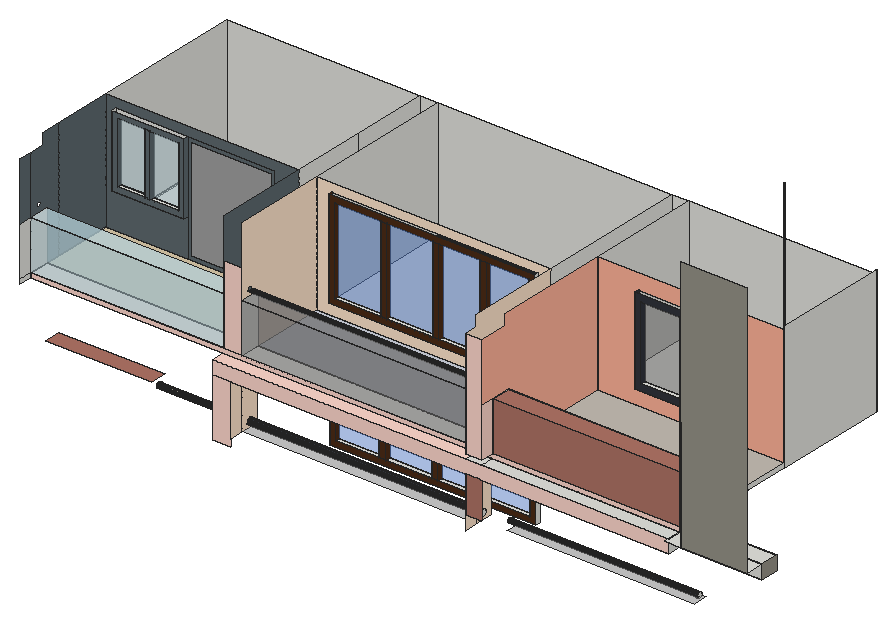
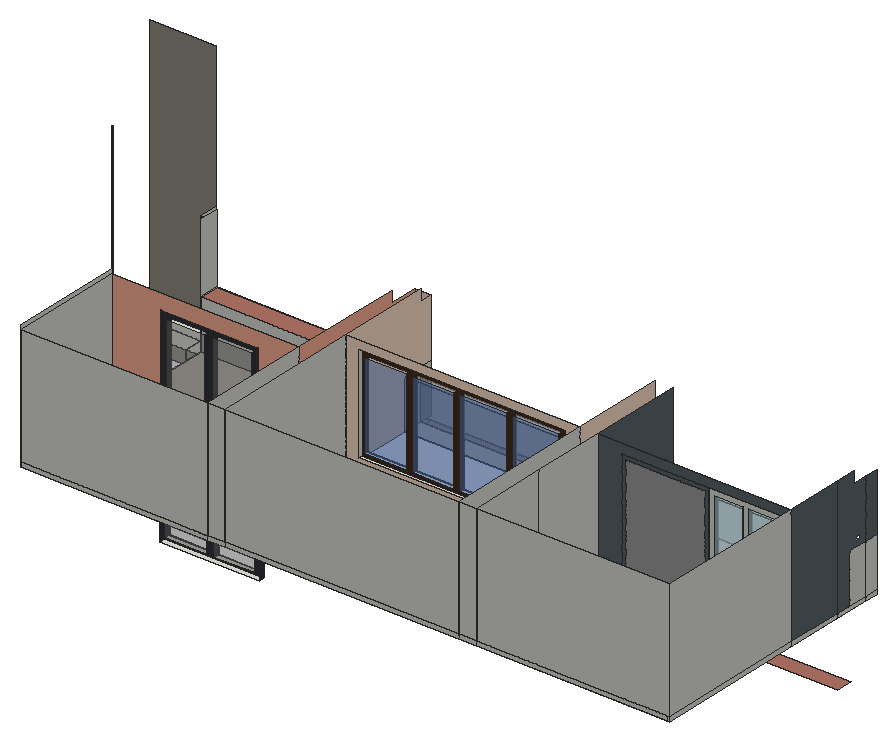
# SketchUp Ruby script. Lengths in inches.
U = 1.inch
M = Sketchup.active_model
def pt(a) = Geom::Point3d.new(a.map { |v| v * U })
def face(e, loops, mat)
  f = e.add_face(loops[0].map { |a| pt(a) })
  loops[1..].each { |l| e.add_face(l.map { |a| pt(a) }).erase! }
  f.material = f.back_material = mat if mat
  f
end
# faces: each face lists its corners as indices into pts; further lists are holes
def faces(e, pts, list, mat = nil) = list.each { |f| face(e, (f[0].is_a?(Array) ? f : [f]).map { |l| l.map { |i| pts[i] } }, mat) }
# xy, xz, yz: faces in a plane at the given z, y or x. An outline is a flat list of corners, or four numbers for a rectangle; further outlines are holes
def ring(l) = l.size == 4 ? [[l[0], l[1]], [l[2], l[1]], [l[2], l[3]], [l[0], l[3]]] : l.each_slice(2).to_a
def flat(e, list, mat, &to3) = list.each { |f| face(e, (f[0].is_a?(Array) ? f : [f]).map { |l| ring(l).map { |u, v| to3.(u, v) } }, mat) }
def xy(e, z, list, mat = nil) = flat(e, list, mat) { |x, y| [x, y, z] }
def xz(e, y, list, mat = nil) = flat(e, list, mat) { |x, z| [x, y, z] }
def yz(e, x, list, mat = nil) = flat(e, list, mat) { |y, z| [x, y, z] }
def lines(e, pts, list) = list.each { |a, b| e.add_line(pt(pts[a]), pt(pts[b])) }
# prism: a flat outline (further loops are holes) pulled along v
def prism(e, loops, v, mat = nil)
  f = face(e, loops, mat); d = Geom::Vector3d.new(v.map { |x| x * U })
  f.pushpull(f.normal.samedirection?(d) ? d.length : -d.length)
end
def box(e, o, s, mat = nil) = prism(e, [[o, [o[0] + s[0], o[1], o[2]], [o[0] + s[0], o[1] + s[1], o[2]], [o[0], o[1] + s[1], o[2]]]], [0, 0, s[2]], mat)
def at(x, y, z, deg = 0) = Geom::Transformation.translation(pt([x, y, z])) * Geom::Transformation.rotation(ORIGIN, Z_AXIS, deg.degrees)
def axes(o, x, y, z) = Geom::Transformation.new([*x, 0, *y, 0, *z, 0, *pt(o).to_a, 1])
def part(name) = M.definitions.add(name)
# library, detail: a bought-in or finely detailed component or shape, given as its bounding box
def library(name, o, s) = part(name).tap { |d| box(d.entities, o, s) }
def detail(e, o, s) = box(e.add_group.entities, o, s)
def put(e, d, t, mat = nil) = e.add_instance(d, t).tap { |i| i.material = mat if mat }
def group(e, t, mat = nil) = e.add_group.tap { |g| g.transformation = t; g.material = mat if mat }.entities
root = M.entities
M.materials.add("[Blinds Vertical Stripe Gray]").color = [160, 160, 160]
M.materials.add("[Color B01]").color = [255, 216, 204]
M.materials.add("[Color B02]").color = [255, 178, 153]
M.materials.add("[Color C01]").color = [255, 229, 204]
M.materials.add("[Field Rectangle Tile]").color = [196, 189, 179]
M.materials.add("[Field Square Tile]").color = [217, 201, 169]
M.materials.add("[Formica Graystone]").color = [149, 146, 135]
M.materials.add("[Formica Laminate Dark]").color = [50, 53, 60]
M.materials.add("[Formica Speckled Grey]").color = [94, 105, 111]
M.materials.add("[Marble Carrara Floor Tile]").color = [204, 208, 219]
M.materials.add("[Stone Flagstone Ashlar]").color = [175, 116, 102]
M.materials.add("[Stone Flagstone Ashlar]1").color = [175, 116, 102]
M.materials.add("[Terrazzo Tile Light]").color = [219, 217, 210]
M.materials.add("[Translucent Glass Blue]").color = [100, 149, 237]
M.materials["[Translucent Glass Blue]"].alpha = 0.5
M.materials.add("[Translucent Glass Gray]").color = [128, 128, 128]
M.materials["[Translucent Glass Gray]"].alpha = 0.5
M.materials.add("[Translucent Glass Safety]").color = [204, 235, 244]
M.materials["[Translucent Glass Safety]"].alpha = 0.5
M.materials.add("[Wood Veneer 01]").color = [76, 44, 23]
xy(root,1479.27,[[1311,1143.68,1873.75,1156.55]])
xy(root,1494.08,[[1325.8125,1143.68,1445.44,1156.55],[1463.27,1143.68,1588.57,1156.55],[1606.39,1143.68,1714.84,1156.55],[1732.67,1143.68,1858.94,1156.55]])
xy(root,1501.65,[[2060.83,1241.24,2333.7,1257.37]])
xy(root,1515.1,[[2074.28,1241.24,2184.97,1257.37],[2204.54,1241.24,2320.25,1257.37]])
xy(root,1576.3125,[[1950.59,950.43,2463.34,950.43,2463.34,954.56,2463.4,992.68,1950.59,992.68]],"[Translucent Glass Gray]")
xy(root,1581.3125,[[1036.41,967.7,1037.9,967.89,1039.29,968.47,1040.48,969.38,1041.39,970.57,1041.96,971.96,1042.16,973.45,1041.96,974.93,1041.39,976.32,1040.48,977.51,1039.29,978.43,1037.9,979,1036.41,979.2,1034.92,979,1033.54,978.43,1032.34,977.51,1031.43,976.32,1030.86,974.93,1030.66,973.45,1030.86,971.96,1031.43,970.57,1032.34,969.38,1033.54,968.47,1034.92,967.89]])
xy(root,1582.25,[[1087.54,967.7,1089.02,967.89,1090.41,968.47,1091.6,969.38,1092.51,970.57,1093.09,971.96,1093.29,973.45,1093.09,974.93,1092.51,976.32,1091.6,977.51,1090.41,978.43,1089.02,979,1087.54,979.2,1086.05,979,1084.66,978.43,1083.47,977.51,1082.56,976.32,1081.98,974.93,1081.79,973.45,1081.98,971.96,1082.56,970.57,1083.47,969.38,1084.66,968.47,1086.05,967.89]])
xy(root,1582.375,[[1142.72,967.7,1144.21,967.89,1145.6,968.47,1146.79,969.38,1147.7,970.57,1148.28,971.96,1148.47,973.45,1148.28,974.93,1147.7,976.32,1146.79,977.51,1145.6,978.43,1144.21,979,1142.72,979.2,1141.23,979,1139.85,978.43,1138.66,977.51,1137.74,976.32,1137.17,974.93,1136.97,973.45,1137.17,971.96,1137.74,970.57,1138.66,969.38,1139.85,968.47,1141.23,967.89]])
xy(root,1582.8125,[[994.85,967.7,996.34,967.89,997.72,968.47,998.91,969.38,999.83,970.57,1000.4,971.96,1000.6,973.45,1000.4,974.93,999.83,976.32,998.91,977.51,997.72,978.43,996.34,979,994.85,979.2,993.36,979,991.97,978.43,990.78,977.51,989.87,976.32,989.29,974.93,989.1,973.45,989.29,971.96,989.87,970.57,990.78,969.38,991.97,968.47,993.36,967.89]])
xy(root,1583.0625,[[1194.79,967.7,1196.27,967.89,1197.66,968.47,1198.85,969.38,1199.76,970.57,1200.34,971.96,1200.54,973.45,1200.34,974.93,1199.76,976.32,1198.85,977.51,1197.66,978.43,1196.27,979,1194.79,979.2,1193.3,979,1191.91,978.43,1190.72,977.51,1189.81,976.32,1189.23,974.93,1189.04,973.45,1189.23,971.96,1189.81,970.57,1190.72,969.38,1191.91,968.47,1193.3,967.89]])
xy(root,1600.3125,[[686.75,950.43,976.71,994.87]],"[Stone Flagstone Ashlar]")
xy(root,1600.3125,[[1263.92,899.87,1905.54,950.43]],"[Translucent Glass Gray]")
xy(root,1722.69,[[2074.28,1241.24,2184.97,1257.37],[2204.54,1241.24,2320.25,1257.37]],"[Formica Laminate Dark]")
xy(root,1736.15,[[2060.83,1241.24,2333.7,1257.37]],"[Formica Laminate Dark]")
xy(root,1737.27,[[1325.8125,1143.68,1445.44,1156.55],[1463.27,1143.68,1588.57,1156.55],[1606.39,1143.68,1714.84,1156.55],[1732.67,1143.68,1858.94,1156.55]],"[Wood Veneer 01]")
xy(root,1739.53,[[1905.54,863.74,1950.59,899.87],[1950.59,863.74,2463.34,899.87],[2507.95,899.87,2688.89,950.43]])
xy(root,1739.53,[[1263.92,899.87,2507.95,950.43]],"[Color B02]")
xy(root,1739.53,[[1263.92,863.74,1905.54,899.87]],"[Color C01]")
xy(root,1752.08,[[1311,1143.68,1873.75,1156.55]])
xy(root,1776.9375,[[2463.34,849.3125,2507.95,899.87],[2507.95,849.3125,2688.89,899.87],[1905.54,863.74,1950.59,899.87],[1950.59,863.74,2463.34,899.87],[1214.63,899.87,1214.63,1156.55,1263.92,1156.55,1263.92,950.43,1905.54,950.43,1905.54,1156.55,1950.59,1156.55,1950.59,950.43,1905.54,950.43,1905.54,899.87],
  [1905.54,899.87,1950.59,950.43],[1950.59,899.87,2463.34,950.43],[2463.34,899.87,2507.95,950.43],[2507.95,899.87,2688.89,950.43],[686.75,1156.55,1214.63,1571.68],
  [1214.63,1156.55,1263.92,1571.68],[1263.92,1156.55,1905.54,1571.68],[1905.54,1156.55,1950.59,1571.68],[1950.59,1257.37,2463.34,1571.68],[2463.34,1257.37,2463.8,1257.37,2464.28,1571.68,2463.34,1571.68],
  [2463.8,1257.37,2464.28,1257.37,2464.28,1571.68]])
xy(root,1776.9375,[[1214.63,863.74,1905.54,899.87]],"[Color B01]")
xy(root,1776.9375,[[1950.59,950.43,2463.34,1156.55],[1950.59,1156.55,2463.34,1257.37]],"[Color B02]")
xy(root,1776.9375,[[1263.92,950.43,1905.54,1156.55]],"[Color C01]")
xy(root,1776.9375,[[686.75,899.87,1214.63,1156.55]],"[Terrazzo Tile Light]")
xy(root,1788.9375,[[1905.54,863.74,1950.59,899.87],[686.75,899.87,1214.63,954.56],[1214.63,899.87,1263.92,1571.68],[1263.92,899.87,1905.54,954.56],[1905.54,899.87,1950.59,1571.68],
  [1950.59,899.87,2463.34,954.56],[686.75,1156.55,692.23,1571.68],[692.23,1156.55,1214.63,1571.68],[1263.92,1156.55,1905.54,1571.68],[1950.59,1258.93,2463.34,1571.68]])
xy(root,1788.9375,[[1950.59,954.56,2463.34,1258.93]],"[Field Rectangle Tile]")
xy(root,1788.9375,[[686.75,954.56,1214.63,1156.55]],"[Field Square Tile]")
xy(root,1788.9375,[[1263.92,954.56,1905.54,1156.55]],"[Marble Carrara Floor Tile]")
xy(root,1824.96,[[1306.61,1144.55,1869.61,1156.55]])
xy(root,1835.7,[[2062.91,1246.93,2329.66,1258.93]])
xy(root,1840.32,[[1321.97,1144.55,1448.68,1156.55],[1465.17,1144.55,1591.81,1156.55],[1608.29,1144.55,1721.62,1156.55],[1738.1,1144.55,1854.25,1156.55]])
xy(root,1853.18,[[2080.39,1246.93,2186.14,1258.93],[2207.95,1246.93,2312.17,1258.93]])
xy(root,1892.5,[[713.49,1144.55,910.11,1156.55]])
xy(root,1906.84,[[727.84,1144.55,801.89,1156.55],[817.41,1144.55,895.77,1156.55]])
xy(root,1923.4375,[[1950.59,899.87,2463.34,954.56]],"[Stone Flagstone Ashlar]")
xy(root,1923.4375,[[1263.92,899.87,1905.54,954.56]],"[Translucent Glass Gray]")
xy(root,1923.4375,[[686.75,899.87,1214.63,954.56]],"[Translucent Glass Safety]")
xz(root,849.3125,[[2507.95,1776.9375,2688.89,2476.875]],"[Formica Graystone]")
xz(root,863.74,[[1214.63,1581.51,1263.92,1739.53],[1214.63,1739.53,2463.34,1776.9375],[1905.54,1788.9375,1950.59,2083.5625]],"[Color B01]")
xz(root,863.74,[[1905.54,1639.44,1950.59,1739.53]],"[Stone Flagstone Ashlar]1")
xz(root,899.87,[[1905.54,1739.53,1950.59,1776.9375],[1950.59,1739.53,2463.34,1776.9375],[2463.34,1739.53,2507.95,1776.9375],[2507.95,1739.53,2688.89,1776.9375]])
xz(root,899.87,[[686.75,1776.9375,2463.34,1788.9375],[2463.34,1776.9375,2507.95,2083.5625],[1214.63,1788.9375,1263.92,2003.5]],"[Color B01]")
xz(root,899.87,[[1950.59,1788.9375,2463.34,1923.4375]],"[Stone Flagstone Ashlar]")
xz(root,899.87,[[1263.92,1788.9375,1905.54,1923.4375]],"[Translucent Glass Gray]")
xz(root,899.87,[[686.75,1788.9375,1214.63,1923.4375]],"[Translucent Glass Safety]")
xz(root,950.43,[[1263.92,1739.53,1905.54,1776.9375],[1905.54,1739.53,1950.59,1776.9375],[1950.59,1739.53,2507.95,1776.9375],[2507.95,1739.53,2688.89,1776.9375]])
xz(root,954.56,[[1950.59,1788.9375,2463.34,1923.4375]])
xz(root,954.56,[[1263.92,1788.9375,1905.54,1923.4375]],"[Translucent Glass Gray]")
xz(root,954.56,[[686.75,1788.9375,1214.63,1923.4375]],"[Translucent Glass Safety]")
xz(root,1143.68,[[[1311,1479.27,1873.75,1752.08],[1325.8125,1494.08,1858.94,1737.27]],[1445.44,1494.08,1463.27,1737.27],[1588.57,1494.08,1606.39,1737.27],[1714.84,1494.08,1732.67,1737.27]],"[Wood Veneer 01]")
xz(root,1144.55,[[[713.49,1892.5,910.11,2089.12],[727.84,1906.84,895.77,2074.78]],[801.89,1906.84,817.41,2074.78]],"[Formica Speckled Grey]")
xz(root,1144.55,[[[1306.61,1824.96,1869.61,2092.65],[1321.97,1840.32,1854.25,2077.28]],[1448.68,1840.32,1465.17,2077.28],[1591.81,1840.32,1608.29,2077.28],[1721.62,1840.32,1738.1,2077.28]],"[Wood Veneer 01]")
xz(root,1156.55,[[[713.49,1892.5,910.11,2089.12],[817.41,1906.84,895.77,2074.78],[727.84,1906.84,801.89,2074.78]]])
xz(root,1156.55,[[921.82,1800.65,1138.65,2077.41]],"[Blinds Vertical Stripe Gray]")
xz(root,1156.55,[[[1263.92,1788.9375,1905.54,2114.125],[1306.61,1824.96,1869.61,2092.65]]],"[Color C01]")
xz(root,1156.55,[[686.75,1788.9375,910.11,1788.9375,910.11,1892.5,713.49,1892.5,713.49,2089.12,1150.35,2089.12,1150.35,1788.9375,1214.63,1788.9375,1214.63,2114.125,686.75,2114.125],[[910.11,1788.9375,1150.35,2089.12],[921.82,1800.65,1138.65,2077.41]]],"[Formica Speckled Grey]")
xz(root,1156.55,[[1325.8125,1494.08,1445.44,1737.27],[1463.27,1494.08,1588.57,1737.27],[1606.39,1494.08,1714.84,1737.27],[1732.67,1494.08,1858.94,1737.27],[1321.97,1840.32,1448.68,2077.28],
  [1465.17,1840.32,1591.81,2077.28],[1608.29,1840.32,1721.62,2077.28],[1738.1,1840.32,1854.25,2077.28]],"[Translucent Glass Blue]")
xz(root,1156.55,[[727.84,1906.84,801.89,2074.78],[817.41,1906.84,895.77,2074.78]],"[Translucent Glass Safety]")
xz(root,1241.24,[[[2060.83,1501.65,2333.7,1736.15],[2074.28,1515.1,2320.25,1722.69]],[2184.97,1515.1,2204.54,1722.69]],"[Formica Laminate Dark]")
xz(root,1246.93,[[[2062.91,1835.7,2329.66,2071.89],[2080.39,1853.18,2312.17,2054.4]],[2186.14,1853.18,2207.95,2054.4]],"[Formica Laminate Dark]")
xz(root,1257.37,[[2463.8,1776.9375,2464.28,2476.875]])
xz(root,1257.37,[[2074.28,1515.1,2184.97,1722.69],[2204.54,1515.1,2320.25,1722.69]],"[Translucent Glass Gray]")
xz(root,1258.93,[[[1950.59,1788.9375,2463.34,2114.125],[2062.91,1835.7,2329.66,2071.89]]],"[Color B02]")
xz(root,1258.93,[[2080.39,1853.18,2186.14,2054.4],[2207.95,1853.18,2312.17,2054.4]],"[Translucent Glass Gray]")
xz(root,1571.68,[[686.75,1776.9375,692.23,1788.9375],[692.23,1776.9375,1214.63,1788.9375],[1214.63,1776.9375,1263.92,1788.9375],[1263.92,1776.9375,1905.54,1788.9375],[1905.54,1776.9375,1950.59,1788.9375],
  [1950.59,1776.9375,2463.34,1788.9375],[2463.34,1776.9375,2464.28,2126.125],[686.75,1788.9375,1214.63,2114.125],[1214.63,1788.9375,1263.92,2114.125],[1263.92,1788.9375,1905.54,2114.125],
  [1905.54,1788.9375,1950.59,2114.125],[1950.59,1788.9375,2463.34,2114.125]])
yz(root,686.75,[[863.74,1776.9375,899.87,1788.9375],[899.87,1776.9375,994.87,1788.9375],[994.87,1776.9375,1156.55,1788.9375],[1156.55,1776.9375,1571.68,1788.9375],[863.74,1788.9375,899.87,1923.4375],
  [899.87,1788.9375,954.56,1923.4375],[1156.55,1788.9375,1571.68,2114.125]])
yz(root,686.75,[[[954.56,1788.9375,994.87,1788.9375,994.87,2114.125,941.93,2114.125,941.93,2083.5625,899.87,2083.5625,899.87,1923.4375,954.56,1923.4375],[927.21,1938.33,925.5,1938.56,923.91,1939.22,922.55,1940.26,921.5,1941.63,920.84,1943.22,920.61,1944.93,920.84,1946.64,921.5,1948.23,922.55,1949.6,923.91,1950.65,925.5,1951.31,927.21,1951.53,928.92,1951.31,930.51,1950.65,931.88,1949.6,932.93,1948.23,933.59,1946.64,933.8125,1944.93,933.59,1943.22,932.93,1941.63,931.88,1940.26,930.51,1939.22,928.92,1938.56]],[994.87,1788.9375,1156.55,2114.125],[863.74,1923.4375,899.87,2083.5625]],"[Formica Speckled Grey]")
yz(root,713.49,[[1144.55,1892.5,1156.55,2089.12]])
yz(root,727.84,[[1144.55,1906.84,1156.55,2074.78]],"[Formica Speckled Grey]")
yz(root,801.89,[[1144.55,1906.84,1156.55,2074.78]],"[Formica Speckled Grey]")
yz(root,817.41,[[1144.55,1906.84,1156.55,2074.78]],"[Formica Speckled Grey]")
yz(root,895.77,[[1144.55,1906.84,1156.55,2074.78]],"[Formica Speckled Grey]")
yz(root,910.11,[[1144.55,1892.5,1156.55,2089.12]],"[Formica Speckled Grey]")
yz(root,976.71,[[973.87,1576.82,972.15,1577.04,970.56,1577.7,969.18,1578.76,968.13,1580.13,967.47,1581.73,967.24,1583.44,967.47,1585.16,968.13,1586.75,969.18,1588.125,970.56,1589.18,972.15,1589.84,973.87,1590.07,975.58,1589.84,977.18,1589.18,978.55,1588.125,979.61,1586.75,980.27,1585.16,980.49,1583.44,980.27,1581.73,979.61,1580.13,978.55,1578.76,977.18,1577.7,975.58,1577.04]])
yz(root,1214.63,[[899.87,1788.9375,954.56,1923.4375],[1156.55,1788.9375,1358.15,2114.125],[1358.15,1788.9375,1571.68,2114.125]])
yz(root,1214.63,[[[954.56,1788.9375,954.56,1923.4375,899.87,1923.4375,899.87,2114.125,1156.55,2114.125,1156.55,1788.9375],[927.21,1938.33,928.92,1938.56,930.51,1939.22,931.88,1940.26,932.93,1941.63,933.59,1943.22,933.8125,1944.93,933.59,1946.64,932.93,1948.23,931.88,1949.6,930.51,1950.65,928.92,1951.31,927.21,1951.53,925.5,1951.31,923.91,1950.65,922.55,1949.6,921.5,1948.23,920.84,1946.64,920.61,1944.93,920.84,1943.22,921.5,1941.63,922.55,1940.26,923.91,1939.22,925.5,1938.56]]],"[Formica Speckled Grey]")
yz(root,1263.92,[[899.87,1788.9375,954.56,1923.4375],[1156.55,1788.9375,1571.68,2114.125]])
yz(root,1263.92,[[863.74,1600.3125,899.87,1739.53],[[899.87,1600.3125,950.43,1739.53],[925.15,1609.2,922.98,1609.48,920.96,1610.32,919.23,1611.65,917.9,1613.39,917.06,1615.41,916.77,1617.57,917.06,1619.74,917.9,1621.76,919.23,1623.5,920.96,1624.83,922.98,1625.66,925.15,1625.95,927.32,1625.66,929.34,1624.83,931.07,1623.5,932.4,1621.76,933.24,1619.74,933.52,1617.57,933.24,1615.41,932.4,1613.39,931.07,1611.65,929.34,1610.32,927.32,1609.48]],[[954.56,1788.9375,1156.55,1788.9375,1156.55,2114.125,899.87,2114.125,899.87,1923.4375,954.56,1923.4375],[927.21,1934.21,925.5,1934.4375,923.9,1935.1,922.53,1936.15,921.48,1937.52,920.8125,1939.12,920.59,1940.84,920.8125,1942.55,921.48,1944.15,922.53,1945.52,923.9,1946.57,925.5,1947.24,927.21,1947.46,928.93,1947.24,930.53,1946.57,931.9,1945.52,932.95,1944.15,933.61,1942.55,933.84,1940.84,933.61,1939.12,932.95,1937.52,931.9,1936.15,930.53,1935.1,928.93,1934.4375]]],"[Color C01]")
yz(root,1306.61,[[1144.55,1824.96,1156.55,2092.65]],"[Wood Veneer 01]")
yz(root,1311,[[1143.68,1479.27,1156.55,1752.08]])
yz(root,1321.97,[[1144.55,1840.32,1156.55,2077.28]],"[Wood Veneer 01]")
yz(root,1325.8125,[[1143.68,1494.08,1156.55,1737.27]],"[Wood Veneer 01]")
yz(root,1445.44,[[1143.68,1494.08,1156.55,1737.27]],"[Wood Veneer 01]")
yz(root,1448.68,[[1144.55,1840.32,1156.55,2077.28]],"[Wood Veneer 01]")
yz(root,1463.27,[[1143.68,1494.08,1156.55,1737.27]],"[Wood Veneer 01]")
yz(root,1465.17,[[1144.55,1840.32,1156.55,2077.28]],"[Wood Veneer 01]")
yz(root,1588.57,[[1143.68,1494.08,1156.55,1737.27]],"[Wood Veneer 01]")
yz(root,1591.81,[[1144.55,1840.32,1156.55,2077.28]],"[Wood Veneer 01]")
yz(root,1606.39,[[1143.68,1494.08,1156.55,1737.27]],"[Wood Veneer 01]")
yz(root,1608.29,[[1144.55,1840.32,1156.55,2077.28]],"[Wood Veneer 01]")
yz(root,1714.84,[[1143.68,1494.08,1156.55,1737.27]],"[Wood Veneer 01]")
yz(root,1721.62,[[1144.55,1840.32,1156.55,2077.28]],"[Wood Veneer 01]")
yz(root,1732.67,[[1143.68,1494.08,1156.55,1737.27]],"[Wood Veneer 01]")
yz(root,1738.1,[[1144.55,1840.32,1156.55,2077.28]],"[Wood Veneer 01]")
yz(root,1854.25,[[1144.55,1840.32,1156.55,2077.28]],"[Wood Veneer 01]")
yz(root,1858.94,[[1143.68,1494.08,1156.55,1737.27]],"[Wood Veneer 01]")
yz(root,1869.61,[[1144.55,1824.96,1156.55,2092.65]])
yz(root,1873.75,[[1143.68,1479.27,1156.55,1752.08]])
yz(root,1905.54,[[925.15,1609.2,927.32,1609.48,929.34,1610.32,931.07,1611.65,932.4,1613.39,933.24,1615.41,933.52,1617.57,933.24,1619.74,932.4,1621.76,931.07,1623.5,929.34,1624.83,927.32,1625.66,925.15,1625.95,922.98,1625.66,920.96,1624.83,919.23,1623.5,917.9,1621.76,917.06,1619.74,916.77,1617.57,917.06,1615.41,917.9,1613.39,919.23,1611.65,920.96,1610.32,922.98,1609.48],[863.74,1788.9375,899.87,1923.4375],[899.87,1788.9375,954.56,1923.4375],[1156.55,1788.9375,1571.68,2114.125],[927.21,1934.21,928.93,1934.4375,930.53,1935.1,931.9,1936.15,932.95,1937.52,933.61,1939.12,933.84,1940.84,933.61,1942.55,932.95,1944.15,931.9,1945.52,930.53,1946.57,928.93,1947.24,927.21,1947.46,925.5,1947.24,923.9,1946.57,922.53,1945.52,921.48,1944.15,920.8125,1942.55,920.59,1940.84,920.8125,1939.12,921.48,1937.52,922.53,1936.15,923.9,1935.1,925.5,1934.4375]])
yz(root,1905.54,[[863.74,1600.3125,899.87,1739.53],[[899.87,1600.3125,950.43,1776.9375],[925.15,1609.2,927.32,1609.48,929.34,1610.32,931.07,1611.65,932.4,1613.39,933.24,1615.41,933.52,1617.57,933.24,1619.74,932.4,1621.76,931.07,1623.5,929.34,1624.83,927.32,1625.66,925.15,1625.95,922.98,1625.66,920.96,1624.83,919.23,1623.5,917.9,1621.76,917.06,1619.74,916.77,1617.57,917.06,1615.41,917.9,1613.39,919.23,1611.65,920.96,1610.32,922.98,1609.48]],[[954.56,1788.9375,954.56,1923.4375,863.74,1923.4375,863.74,2083.5625,899.87,2083.5625,899.87,2114.125,1156.55,2114.125,1156.55,1788.9375],[927.21,1934.21,928.93,1934.4375,930.53,1935.1,931.9,1936.15,932.95,1937.52,933.61,1939.12,933.84,1940.84,933.61,1942.55,932.95,1944.15,931.9,1945.52,930.53,1946.57,928.93,1947.24,927.21,1947.46,925.5,1947.24,923.9,1946.57,922.53,1945.52,921.48,1944.15,920.8125,1942.55,920.59,1940.84,920.8125,1939.12,921.48,1937.52,922.53,1936.15,923.9,1935.1,925.5,1934.4375]]],"[Color C01]")
yz(root,1950.59,[[899.87,1788.9375,954.56,1923.4375],[1258.93,1788.9375,1571.68,2114.125]])
yz(root,1950.59,[[863.74,1788.9375,899.87,1923.4375]],"[Color B01]")
yz(root,1950.59,[[954.56,1788.9375,1258.93,1788.9375,1258.93,2114.125,941.93,2114.125,941.93,2083.5625,863.74,2083.5625,863.74,1923.4375,954.56,1923.4375]],"[Color B02]")
yz(root,2060.83,[[1241.24,1501.65,1257.37,1736.15]],"[Formica Laminate Dark]")
yz(root,2062.91,[[1246.93,1835.7,1258.93,2071.89]],"[Formica Laminate Dark]")
yz(root,2074.28,[[1241.24,1515.1,1257.37,1722.69]],"[Formica Laminate Dark]")
yz(root,2080.39,[[1246.93,1853.18,1258.93,2054.4]],"[Formica Laminate Dark]")
yz(root,2184.97,[[1241.24,1515.1,1257.37,1722.69]],"[Formica Laminate Dark]")
yz(root,2186.14,[[1246.93,1853.18,1258.93,2054.4]],"[Formica Laminate Dark]")
yz(root,2204.54,[[1241.24,1515.1,1257.37,1722.69]],"[Formica Laminate Dark]")
yz(root,2207.95,[[1246.93,1853.18,1258.93,2054.4]],"[Formica Laminate Dark]")
yz(root,2312.17,[[1246.93,1853.18,1258.93,2054.4]],"[Formica Laminate Dark]")
yz(root,2320.25,[[1241.24,1515.1,1257.37,1722.69]],"[Formica Laminate Dark]")
yz(root,2329.66,[[1246.93,1835.7,1258.93,2071.89]],"[Formica Laminate Dark]")
yz(root,2333.7,[[1241.24,1501.65,1257.37,1736.15]],"[Formica Laminate Dark]")
yz(root,2463.34,[[863.74,1739.53,899.87,1776.9375],[899.87,1776.9375,954.56,1788.9375],[954.56,1776.9375,1571.68,1788.9375],[899.87,1788.9375,954.56,1923.4375],[1258.93,1788.9375,1571.68,2114.125],
  [899.87,1923.4375,954.56,2114.125]])
yz(root,2464.28,[[1257.37,1776.9375,1257.37,2476.875,1258.05,2476.875,1258.05,2126.125,1571.68,2126.125,1571.68,1776.9375]])
yz(root,2507.95,[[899.87,1739.53,950.43,1776.9375],[849.3125,1776.9375,899.87,2083.5625]])
yz(root,2688.89,[[899.87,1739.53,950.43,1776.9375]],"[Formica Graystone]")
p = [[976.71,972.15,1577.04],[976.71,973.87,1576.82],[1214.63,973.87,1576.82],[1214.63,972.15,1577.04],[976.71,975.58,1577.04],[1214.63,975.58,1577.04],
  [976.71,970.56,1577.7],[1214.63,970.56,1577.7],[976.71,977.18,1577.7],[1214.63,977.18,1577.7],[976.71,969.18,1578.76],[1214.63,969.18,1578.76],
  [976.71,978.55,1578.76],[1214.63,978.55,1578.76],[976.71,968.13,1580.13],[1214.63,968.13,1580.13],[976.71,979.61,1580.13],[1214.63,979.61,1580.13],
  [976.71,967.47,1581.73],[1214.63,967.47,1581.73],[976.71,980.27,1581.73],[1214.63,980.27,1581.73],[976.71,967.24,1583.44],[1214.63,967.24,1583.44],
  [976.71,980.49,1583.44],[1214.63,980.49,1583.44],[976.71,967.47,1585.16],[1214.63,967.47,1585.16],[976.71,980.27,1585.16],[1214.63,980.27,1585.16],
  [976.71,968.13,1586.75],[1214.63,968.13,1586.75],[976.71,979.61,1586.75],[1214.63,979.61,1586.75],[2463.35,962.98,1592.2],[2463.36,963.19,1590.63],
  [2463.36,963.8,1589.17],[2463.36,964.76,1587.92],[2463.36,966.01,1586.95],[2463.36,967.48,1586.35],[2463.36,969.05,1586.14],[2463.37,970.61,1586.35],
  [2463.37,972.08,1586.95],[2463.37,973.33,1587.92],[2463.37,974.3,1589.17],[2463.375,974.9,1590.63],[2463.375,975.11,1592.2],[2463.375,974.9,1593.77],
  [2463.37,974.3,1595.23],[2463.37,973.33,1596.49],[2463.37,972.08,1597.45],[2463.37,970.61,1598.06],[2463.36,969.05,1598.27],[2463.36,967.48,1598.06],
  [2463.36,966.01,1597.45],[2463.36,964.76,1596.49],[2463.36,963.8,1595.23],[2463.36,963.19,1593.77],[1941.67,963.98,1590.63],[1941.67,963.78,1592.2],
  [1941.67,963.98,1593.77],[1941.67,964.59,1595.23],[1941.67,965.55,1596.49],[1941.67,966.81,1597.45],[1941.67,968.27,1598.06],[1941.68,969.84,1598.27],
  [1941.68,971.41,1598.06],[1941.68,972.87,1597.45],[1941.68,974.125,1596.49],[1941.69,975.09,1595.23],[1941.6875,975.69,1593.77],[1941.6875,975.9,1592.2],
  [1941.6875,975.69,1590.63],[1941.69,975.09,1589.17],[1941.68,974.125,1587.92],[1941.68,972.87,1586.95],[1941.68,971.41,1586.35],[1941.68,969.84,1586.14],
  [1941.67,968.27,1586.35],[1941.67,966.81,1586.95],[1941.67,965.55,1587.92],[1941.67,964.59,1589.17],[976.71,969.18,1588.125],[1214.63,969.18,1588.125],
  [976.71,978.55,1588.125],[1214.63,978.55,1588.125],[976.71,970.56,1589.18],[1214.63,970.56,1589.18],[976.71,977.18,1589.18],[1214.63,977.18,1589.18],
  [976.71,972.15,1589.84],[1214.63,972.15,1589.84],[976.71,975.58,1589.84],[1214.63,975.58,1589.84],[976.71,973.87,1590.07],[1214.63,973.87,1590.07],
  [1905.54,925.15,1609.2],[1905.54,922.98,1609.48],[1263.92,922.98,1609.48],[1263.92,925.15,1609.2],[1905.54,927.32,1609.48],[1263.92,927.32,1609.48],
  [1905.54,920.96,1610.32],[1263.92,920.96,1610.32],[1905.54,929.34,1610.32],[1263.92,929.34,1610.32],[1905.54,919.23,1611.65],[1263.92,919.23,1611.65],
  [1905.54,931.07,1611.65],[1263.92,931.07,1611.65],[1905.54,917.9,1613.39],[1263.92,917.9,1613.39],[1905.54,932.4,1613.39],[1263.92,932.4,1613.39],
  [1905.54,917.06,1615.41],[1263.92,917.06,1615.41],[1905.54,933.24,1615.41],[1263.92,933.24,1615.41],[1905.54,916.77,1617.57],[1263.92,916.77,1617.57],
  [1905.54,933.52,1617.57],[1263.92,933.52,1617.57],[1905.54,917.06,1619.74],[1263.92,917.06,1619.74],[1905.54,933.24,1619.74],[1263.92,933.24,1619.74],
  [1905.54,917.9,1621.76],[1263.92,917.9,1621.76],[1905.54,932.4,1621.76],[1263.92,932.4,1621.76],[1905.54,919.23,1623.5],[1263.92,919.23,1623.5],
  [1905.54,931.07,1623.5],[1263.92,931.07,1623.5],[1905.54,920.96,1624.83],[1263.92,920.96,1624.83],[1905.54,929.34,1624.83],[1263.92,929.34,1624.83],
  [1905.54,922.98,1625.66],[1263.92,922.98,1625.66],[1905.54,927.32,1625.66],[1263.92,927.32,1625.66],[1905.54,925.15,1625.95],[1263.92,925.15,1625.95],
  [1905.54,927.21,1934.21],[1905.54,925.5,1934.4375],[1263.92,925.5,1934.4375],[1263.92,927.21,1934.21],[1905.54,928.93,1934.4375],[1263.92,928.93,1934.4375],
  [1905.54,923.9,1935.1],[1263.92,923.9,1935.1],[1905.54,930.53,1935.1],[1263.92,930.53,1935.1],[1905.54,922.53,1936.15],[1263.92,922.53,1936.15],
  [1905.54,931.9,1936.15],[1263.92,931.9,1936.15],[1905.54,921.48,1937.52],[1263.92,921.48,1937.52],[1905.54,932.95,1937.52],[1263.92,932.95,1937.52],
  [1905.54,920.8125,1939.12],[1263.92,920.8125,1939.12],[1905.54,933.61,1939.12],[1263.92,933.61,1939.12]]
faces(root,p,[[0,1,2,3],[1,4,5,2],[6,0,3,7],[4,8,9,5],[10,6,7,11],[8,12,13,9],[14,10,11,15],[12,16,17,13],
  [18,14,15,19],[16,20,21,17],[22,18,19,23],[20,24,25,21],[26,22,23,27],[24,28,29,25],[30,26,27,31],[28,32,33,29],
  [82,30,31,83],[32,84,85,33],[86,82,83,87],[84,88,89,85],[90,86,87,91],[88,92,93,89],[94,90,91,95],[92,94,95,93]],"[Formica Graystone]")
faces(root,p,[[34,35,36,37,38,39,40,41,42,43,44,45,46,47,48,49,50,51,52,53,54,55,56,57],[58,59,60,61,62,63,64,65,66,67,68,69,70,71,72,73,74,75,76,77,78,79,80,81]])
faces(root,p,[[40,39,78,77],[41,40,77,76],[39,38,79,78],[42,41,76,75],[38,37,80,79],[43,42,75,74],[37,36,81,80],[44,43,74,73],
  [36,35,58,81],[45,44,73,72],[35,34,59,58],[46,45,72,71],[34,57,60,59],[47,46,71,70],[57,56,61,60],[48,47,70,69],
  [56,55,62,61],[49,48,69,68],[55,54,63,62],[50,49,68,67],[54,53,64,63],[51,50,67,66],[53,52,65,64],[52,51,66,65],
  [96,97,98,99],[100,96,99,101],[97,102,103,98],[104,100,101,105],[102,106,107,103],[108,104,105,109],[106,110,111,107],[112,108,109,113],
  [110,114,115,111],[116,112,113,117],[114,118,119,115],[120,116,117,121],[118,122,123,119],[124,120,121,125],[122,126,127,123],[128,124,125,129],
  [126,130,131,127],[132,128,129,133],[130,134,135,131],[136,132,133,137],[134,138,139,135],[140,136,137,141],[138,142,143,139],[142,140,141,143],
  [144,145,146,147],[148,144,147,149],[145,150,151,146],[152,148,149,153],[150,154,155,151],[156,152,153,157],[154,158,159,155],[160,156,157,161],
  [158,162,163,159],[164,160,161,165]],"[Formica Laminate Dark]")
